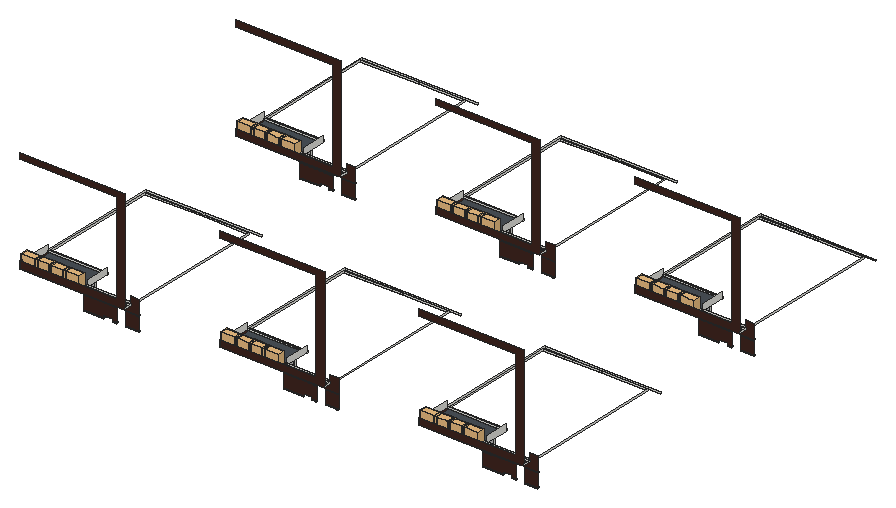
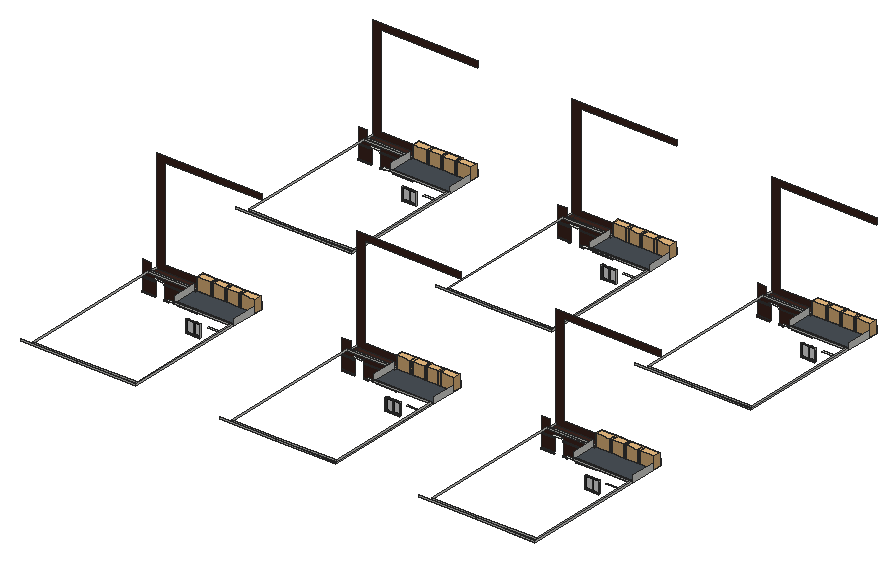
# SketchUp Ruby script. Lengths in inches.
U = 1.inch
M = Sketchup.active_model
def pt(a) = Geom::Point3d.new(a.map { |v| v * U })
def face(e, loops, mat)
  f = e.add_face(loops[0].map { |a| pt(a) })
  loops[1..].each { |l| e.add_face(l.map { |a| pt(a) }).erase! }
  f.material = f.back_material = mat if mat
  f
end
# faces: each face lists its corners as indices into pts; further lists are holes
def faces(e, pts, list, mat = nil) = list.each { |f| face(e, (f[0].is_a?(Array) ? f : [f]).map { |l| l.map { |i| pts[i] } }, mat) }
# xy, xz, yz: faces in a plane at the given z, y or x. An outline is a flat list of corners, or four numbers for a rectangle; further outlines are holes
def ring(l) = l.size == 4 ? [[l[0], l[1]], [l[2], l[1]], [l[2], l[3]], [l[0], l[3]]] : l.each_slice(2).to_a
def flat(e, list, mat, &to3) = list.each { |f| face(e, (f[0].is_a?(Array) ? f : [f]).map { |l| ring(l).map { |u, v| to3.(u, v) } }, mat) }
def xy(e, z, list, mat = nil) = flat(e, list, mat) { |x, y| [x, y, z] }
def xz(e, y, list, mat = nil) = flat(e, list, mat) { |x, z| [x, y, z] }
def yz(e, x, list, mat = nil) = flat(e, list, mat) { |y, z| [x, y, z] }
def lines(e, pts, list) = list.each { |a, b| e.add_line(pt(pts[a]), pt(pts[b])) }
# prism: a flat outline (further loops are holes) pulled along v
def prism(e, loops, v, mat = nil)
  f = face(e, loops, mat); d = Geom::Vector3d.new(v.map { |x| x * U })
  f.pushpull(f.normal.samedirection?(d) ? d.length : -d.length)
end
def box(e, o, s, mat = nil) = prism(e, [[o, [o[0] + s[0], o[1], o[2]], [o[0] + s[0], o[1] + s[1], o[2]], [o[0], o[1] + s[1], o[2]]]], [0, 0, s[2]], mat)
def at(x, y, z, deg = 0) = Geom::Transformation.translation(pt([x, y, z])) * Geom::Transformation.rotation(ORIGIN, Z_AXIS, deg.degrees)
def axes(o, x, y, z) = Geom::Transformation.new([*x, 0, *y, 0, *z, 0, *pt(o).to_a, 1])
def part(name) = M.definitions.add(name)
# library, detail: a bought-in or finely detailed component or shape, given as its bounding box
def library(name, o, s) = part(name).tap { |d| box(d.entities, o, s) }
def detail(e, o, s) = box(e.add_group.entities, o, s)
def put(e, d, t, mat = nil) = e.add_instance(d, t).tap { |i| i.material = mat if mat }
def group(e, t, mat = nil) = e.add_group.tap { |g| g.transformation = t; g.material = mat if mat }.entities
root = M.entities
M.materials.add("Glass_Tinted_Gray").color = [0, 0, 0]
M.materials["Glass_Tinted_Gray"].alpha = 0.125
M.materials.add("[0043_SaddleBrown]").color = [63, 38, 31]
M.materials.add("[0135_DarkGray]").color = [81, 81, 81]
M.materials.add("[Formica Blue]").color = [73, 80, 86]
M.materials.add("[Mirror 02]").color = [229, 229, 229]
M.materials.add("[Terrazzo Light Blue]").color = [196, 214, 227]
c1 = part("PENTEK_RP Fineline 50S_Sliding_DoorCase_E1")
box(c1.entities,[0,0,0],[1.51,3.66,99.27],"[0135_DarkGray]")
c2 = part("PENTEK_RP Fineline 50S_SlidingDooe_Case_E2")
box(c2.entities,[0,0,0],[96.25,3.66,1.51],"[0135_DarkGray]")
c3 = part("pentek_RP Fineline 50S_SlidingDoor_Case")
put(c3.entities,c1,at(97.76,0,0))
put(c3.entities,c2,at(1.51,0,0))
put(c3.entities,c1,at(0,0,0))
put(c3.entities,c2,at(1.51,0,97.76))
c4 = part("PENTEK_RP Fineline 50S_SlidingDoor_GlazingBead_2")
box(c4.entities,[0,0,0],[0.56,0.59,94.39],"[0135_DarkGray]")
c5 = part("PENTEK_RP Fineline 50S_SlidingDoor_Glass")
box(c5.entities,[0,0,0],[46.58,0.16,94.39],"Glass_Tinted_Gray")
c6 = part("PENTEK_RP Fineline 50S_SlidingDoor_GlazingBead")
box(c6.entities,[0,0,0],[45.47,0.59,0.56],"[0135_DarkGray]")
c7 = part("PENTEK_RP Fineline 50S_SlidingDoor_Leaf_E1")
xy(c7.entities,0,[[0,0,0.93,1.97],[0.93,1.57,1.49,1.97]],"[0135_DarkGray]")
xy(c7.entities,96.25,[[0,0,0.93,0,0.93,1.57,1.49,1.57,1.49,1.97,0,1.97]],"[0135_DarkGray]")
xz(c7.entities,0,[[0,0,0.93,96.25]],"[0135_DarkGray]")
xz(c7.entities,1.57,[[0.93,0,1.49,95.32],[0.93,95.32,1.49,96.25]],"[0135_DarkGray]")
xz(c7.entities,1.97,[[0,0,1.49,96.25]],"[0135_DarkGray]")
yz(c7.entities,0,[[0,0,1.97,96.25]],"[0135_DarkGray]")
yz(c7.entities,0.93,[[0,0,1.57,0.93],[0,0.93,1.57,95.32],[0,95.32,1.57,96.25]],"[0135_DarkGray]")
yz(c7.entities,1.49,[[1.57,0,1.97,95.32],[1.57,95.32,1.97,96.25]],"[0135_DarkGray]")
c8 = part("PENTEK_RP Fineline 50S_SlidingDoor_Leaf_E2")
xy(c8.entities,0,[[0,0,0,1.57,0.56,1.57,0.56,1.97,46.02,1.97,46.02,1.57,46.58,1.57,46.58,0]],"[0135_DarkGray]")
xy(c8.entities,0.93,[[0,0,46.58,1.57]],"[0135_DarkGray]")
xy(c8.entities,1.49,[[0.56,1.57,46.02,1.97]],"[0135_DarkGray]")
xz(c8.entities,0,[[0,0,46.58,0.93]],"[0135_DarkGray]")
xz(c8.entities,1.57,[[0,0,0.56,0.93],[46.02,0,46.58,0.93],[0.56,0.93,46.02,1.49]],"[0135_DarkGray]")
xz(c8.entities,1.97,[[0.56,0,46.02,1.49]],"[0135_DarkGray]")
yz(c8.entities,0,[[0,0,1.57,0.93]],"[0135_DarkGray]")
yz(c8.entities,0.56,[[1.57,0,1.97,0.93],[1.57,0.93,1.97,1.49]],"[0135_DarkGray]")
yz(c8.entities,46.02,[[1.57,0,1.97,0.93],[1.57,0.93,1.97,1.49]],"[0135_DarkGray]")
yz(c8.entities,46.58,[[0,0,1.57,0.93]],"[0135_DarkGray]")
c9 = part("PENTEK_RP Fineline S_SlidingDoor_Leaf1")
put(c9.entities,c4,at(0.93,0,0.93))
put(c9.entities,c4,at(46.96,0,0.93))
put(c9.entities,c5,at(1.49,1.42,0.93))
put(c9.entities,c6,at(1.49,0,0.93))
put(c9.entities,c5,at(1.49,0.59,0.93),"[Terrazzo Light Blue]")
put(c9.entities,c7,at(0,0,0))
put(c9.entities,c7,axes([48.44,0,0],[-1,0,0],[0,1,0],[0,0,1]))
put(c9.entities,c8,axes([0.93,0,96.25],[1,0,0],[0,1,0],[0,0,-1]))
put(c9.entities,c8,at(0.93,0,0))
put(c9.entities,c6,at(1.49,0,94.77))
c10 = part("PENTEK_RP Fineline 50S_SlidingDoor_Leaf2")
put(c10.entities,c5,at(1.49,1.42,0.93))
put(c10.entities,c6,at(1.49,0,94.77))
put(c10.entities,c4,at(46.96,0,0.93))
put(c10.entities,c5,at(1.49,0.59,0.93),"[Mirror 02]")
put(c10.entities,c4,at(0.93,0,0.93))
put(c10.entities,c7,at(0,0,0))
put(c10.entities,c7,axes([48.44,0,0],[-1,0,0],[0,1,0],[0,0,1]))
put(c10.entities,c6,at(1.49,0,0.93))
put(c10.entities,c8,axes([0.93,0,96.25],[1,0,0],[0,1,0],[0,0,-1]))
put(c10.entities,c8,at(0.93,0,0))
c11 = part("PENTEK - Slimmest Steel Sliding Door / Window\#1")
put(c11.entities,c3,at(0,-1.88,-0.09))
put(c11.entities,c9,at(1.51,-2.27,1.42))
put(c11.entities,c10,at(49.32,-0.3,1.42))
c12 = library("Group13",[-203.48,36.63,0],[29.68,67.31,50.64])
xy(root,298.0625,[[258.09,535.375,309.84,540.48],[982.53,535.375,1034.28,540.48],[1706.96,535.375,1758.71,540.48],[258.09,1515.73,309.84,1520.83],[982.53,1515.73,1034.28,1520.83],
  [1706.96,1515.73,1758.71,1520.83]])
xy(root,303,[[348.1875,438.72,419.76,441.04],[451.01,438.72,467.3,441.04],[1072.625,438.72,1144.2,441.04],[1175.45,438.72,1191.74,441.04],[1797.0625,438.72,1868.64,441.04],
  [1899.89,438.72,1916.17,441.04],[500.42,438.73,547.05,441.04],[1224.86,438.73,1271.49,441.04],[1949.3,438.73,1995.93,441.04],[348.1875,1419.07,419.76,1421.39],
  [451.01,1419.07,467.3,1421.39],[1072.625,1419.07,1144.2,1421.39],[1175.45,1419.07,1191.74,1421.39],[1797.0625,1419.07,1868.64,1421.39],[1899.89,1419.07,1916.17,1421.39],
  [500.42,1419.08,547.05,1421.39],[1224.86,1419.08,1271.49,1421.39],[1949.3,1419.08,1995.93,1421.39]])
xy(root,306.15,[[348.1875,438.72,419.76,441.04],[1072.625,438.72,1144.2,441.04],[1797.0625,438.72,1868.64,441.04],[348.1875,1419.07,348.1875,1421.39,419.76,1421.39,419.76,1419.08],[1072.625,1419.07,1072.625,1421.39,1144.2,1421.39,1144.2,1419.08],
  [1797.0625,1419.07,1797.0625,1421.39,1868.64,1421.39,1868.64,1419.08]])
xy(root,306.7,[[547.05,438.72,500.42,438.73,500.42,441.04,547.05,441.04],[1271.49,438.72,1224.86,438.73,1224.86,441.04,1271.49,441.04],[1995.93,438.72,1949.3,438.73,1949.3,441.04,1995.93,441.04],[547.05,1419.07,500.42,1419.08,500.42,1421.39,547.05,1421.39],[1271.49,1419.07,1224.86,1419.08,1224.86,1421.39,1271.49,1421.39],
  [1995.93,1419.07,1949.3,1419.08,1949.3,1421.39,1995.93,1421.39]])
xy(root,306.93,[[451.01,438.72,467.3,441.04],[1175.45,438.72,1191.74,441.04],[1899.89,438.72,1916.17,441.04],[451.01,1419.07,467.3,1421.39],[1175.45,1419.07,1191.74,1421.39],
  [1899.89,1419.07,1916.17,1421.39]])
xy(root,312.4,[[419.76,438.72,451.01,447.84],[1144.2,438.72,1175.45,447.84],[1868.64,438.72,1899.89,447.84],[419.76,1419.07,451.01,1428.19],[1144.2,1419.07,1175.45,1428.19],
  [1868.64,1419.07,1899.89,1428.19]])
xy(root,342.25,[[183.3,535.375,231.3,540.48],[258.09,535.375,309.84,540.48],[907.74,535.375,955.74,540.48],[982.53,535.375,1034.28,540.48],[1632.17,535.375,1680.17,540.48],
  [1706.96,535.375,1758.71,540.48],[183.3,1515.73,231.3,1520.83],[258.09,1515.73,309.84,1520.83],[907.74,1515.73,955.74,1520.83],[982.53,1515.73,1034.28,1520.83],
  [1632.17,1515.73,1680.17,1520.83],[1706.96,1515.73,1758.71,1520.83]])
xy(root,354.05,[[348.1875,438.72,467.3,441.04],[1072.625,438.72,1191.74,441.04],[1797.0625,438.72,1916.17,441.04],[348.1875,1419.07,467.3,1421.39],[1072.625,1419.07,1191.74,1421.39],
  [1797.0625,1419.07,1916.17,1421.39]])
xy(root,354.27,[[547.05,438.72,547.05,441.04,500.42,441.04,500.42,438.73],[1271.49,438.72,1271.49,441.04,1224.86,441.04,1224.86,438.73],[1995.93,438.72,1995.93,441.04,1949.3,441.04,1949.3,438.73],[547.05,1419.07,547.05,1421.39,500.42,1421.39,500.42,1419.08],[1271.49,1419.07,1271.49,1421.39,1224.86,1421.39,1224.86,1419.08],
  [1995.93,1419.07,1995.93,1421.39,1949.3,1421.39,1949.3,1419.08]])
xy(root,355.72,[[348.1875,438.72,467.3,441.04],[1072.625,438.72,1191.74,441.04],[1797.0625,438.72,1916.17,441.04],[348.1875,1419.07,467.3,1421.39],[1072.625,1419.07,1191.74,1421.39],
  [1797.0625,1419.07,1916.17,1421.39]])
xy(root,357.3,[[500.42,438.73,547.05,441.04],[1224.86,438.73,1271.49,441.04],[1949.3,438.73,1995.93,441.04],[500.42,1419.08,547.05,1421.39],[1224.86,1419.08,1271.49,1421.39],
  [1949.3,1419.08,1995.93,1421.39]])
xy(root,365.23,[[467.3,438.72,500.42,447.84],[1191.74,438.72,1224.86,447.84],[1916.17,438.72,1949.3,447.84],[467.3,1419.07,500.42,1428.19],[1191.74,1419.07,1224.86,1428.19],
  [1916.17,1419.07,1949.3,1428.19]])
xy(root,378.25,[[348.1875,438.72,353.97,447.84],[1072.625,438.72,1078.41,447.84],[1797.0625,438.72,1802.84,447.84],[137.5,535.375,137.5,980.35,353.97,980.35,353.97,971.23,144.84,965.96,144.84,540.48,353.97,540.48,353.97,535.375],[861.9375,535.375,861.9375,980.35,1078.41,980.35,1078.41,971.23,869.28,965.96,869.28,540.48,1078.41,540.48,1078.41,535.375],
  [1586.375,535.375,1586.375,980.35,1802.84,980.35,1802.84,971.23,1593.72,965.96,1593.72,540.48,1802.84,540.48,1802.84,535.375],[348.1875,1419.07,353.97,1428.19],[1072.625,1419.07,1078.41,1428.19],[1797.0625,1419.07,1802.84,1428.19],[137.5,1515.73,137.5,1960.7,353.97,1960.7,353.97,1951.58,144.84,1946.3125,144.84,1520.83,353.97,1520.83,353.97,1515.73],
  [861.9375,1515.73,861.9375,1960.7,1078.41,1960.7,1078.41,1951.58,869.28,1946.3125,869.28,1520.83,1078.41,1520.83,1078.41,1515.73],[1586.375,1515.73,1586.375,1960.7,1802.84,1960.7,1802.84,1951.58,1593.72,1946.3125,1593.72,1520.83,1802.84,1520.83,1802.84,1515.73]])
xy(root,378.25,[[137.5,412.04,137.5,535.375,144.5,535.375,144.5,438.72,504.5,438.72,504.5,412.04],[504.5,412.04,517.3125,438.72],[861.9375,412.04,861.9375,535.375,868.9375,535.375,868.9375,438.72,1228.9375,438.72,1228.9375,412.04],[1228.9375,412.04,1241.75,438.72],[1586.375,412.04,1586.375,535.375,1593.375,535.375,1593.375,438.72,1953.375,438.72,1953.375,412.04],
  [1953.375,412.04,1966.1875,438.72],[137.5,1392.39,137.5,1515.73,144.5,1515.73,144.5,1419.07,504.5,1419.07,504.5,1392.39],[504.5,1392.39,517.3125,1419.07],[861.9375,1392.39,861.9375,1515.73,868.9375,1515.73,868.9375,1419.07,1228.9375,1419.07,1228.9375,1392.39],[1228.9375,1392.39,1241.75,1419.07],
  [1586.375,1392.39,1586.375,1515.73,1593.375,1515.73,1593.375,1419.07,1953.375,1419.07,1953.375,1392.39],[1953.375,1392.39,1966.1875,1419.07]],"[0043_SaddleBrown]")
xy(root,378.25,[[144.5,438.72,144.5,535.375,353.97,535.375,353.97,447.84,348.1875,447.84,348.1875,438.72],[868.9375,438.72,868.9375,535.375,1078.41,535.375,1078.41,447.84,1072.625,447.84,1072.625,438.72],[1593.375,438.72,1593.375,535.375,1802.84,535.375,1802.84,447.84,1797.0625,447.84,1797.0625,438.72],[144.5,1419.07,144.5,1515.73,353.97,1515.73,353.97,1428.19,348.1875,1428.19,348.1875,1419.07],[868.9375,1419.07,868.9375,1515.73,1078.41,1515.73,1078.41,1428.19,1072.625,1428.19,1072.625,1419.07],
  [1593.375,1419.07,1593.375,1515.73,1802.84,1515.73,1802.84,1428.19,1797.0625,1428.19,1797.0625,1419.07]],"[Formica Blue]")
xz(root,412.04,[[137.5,378.25,517.3125,378.25,517.3125,755.5,137.5,755.5,137.5,733.125,487.0625,733.125,487.0625,401.6875,137.5,401.6875],[861.9375,378.25,1241.75,378.25,1241.75,755.5,861.9375,755.5,861.9375,733.125,1211.5,733.125,1211.5,401.6875,861.9375,401.6875],[1586.375,378.25,1966.1875,378.25,1966.1875,755.5,1586.375,755.5,1586.375,733.125,1935.9375,733.125,1935.9375,401.6875,1586.375,401.6875]],"[0043_SaddleBrown]")
xz(root,438.72,[[348.1875,378.25,353.97,384.25],[353.97,378.25,504.5,384.25],[504.5,378.25,517.3125,384.25],[1072.625,378.25,1078.41,384.25],[1078.41,378.25,1228.9375,384.25],
  [1228.9375,378.25,1241.75,384.25],[1797.0625,378.25,1802.84,384.25],[1802.84,378.25,1953.375,384.25],[1953.375,378.25,1966.1875,384.25]])
xz(root,438.72,[[348.1875,306.15,419.76,306.15,419.76,312.4,451.01,312.4,451.01,306.93,467.3,306.93,467.3,354.05,348.1875,354.05],[1072.625,306.15,1144.2,306.15,1144.2,312.4,1175.45,312.4,1175.45,306.93,1191.74,306.93,1191.74,354.05,1072.625,354.05],[1797.0625,306.15,1868.64,306.15,1868.64,312.4,1899.89,312.4,1899.89,306.93,1916.17,306.93,1916.17,354.05,1797.0625,354.05]],"[0043_SaddleBrown]")
xz(root,441.04,[[348.1875,303,419.76,306.15],[451.01,303,467.3,306.93],[500.42,303,547.05,306.7],[1072.625,303,1144.2,306.15],[1175.45,303,1191.74,306.93],
  [1224.86,303,1271.49,306.7],[1797.0625,303,1868.64,306.15],[1899.89,303,1916.17,306.93],[1949.3,303,1995.93,306.7],[348.1875,354.05,467.3,355.72],
  [1072.625,354.05,1191.74,355.72],[1797.0625,354.05,1916.17,355.72],[500.42,354.27,547.05,357.3],[1224.86,354.27,1271.49,357.3],[1949.3,354.27,1995.93,357.3]],"[0043_SaddleBrown]")
xz(root,447.84,[[348.1875,378.25,353.97,384.25],[353.97,378.25,521.63,384.25],[1072.625,378.25,1078.41,384.25],[1078.41,378.25,1246.07,384.25],[1797.0625,378.25,1802.84,384.25],
  [1802.84,378.25,1970.51,384.25]])
xz(root,535.375,[[137.5,378.25,353.97,384.25],[861.9375,378.25,1078.41,384.25],[1586.375,378.25,1802.84,384.25]])
xz(root,540.48,[[144.84,378.25,353.97,384.25],[869.28,378.25,1078.41,384.25],[1593.72,378.25,1802.84,384.25]])
xz(root,971.23,[[353.97,378.25,521.63,384.25],[1078.41,378.25,1246.07,384.25],[1802.84,378.25,1970.51,384.25]])
xz(root,980.35,[[137.5,378.25,353.97,384.25],[353.97,378.25,558.625,384.25],[861.9375,378.25,1078.41,384.25],[1078.41,378.25,1283.0625,384.25],[1586.375,378.25,1802.84,384.25],
  [1802.84,378.25,2007.5,384.25]])
xz(root,1392.39,[[137.5,378.25,517.3125,378.25,517.3125,755.5,137.5,755.5,137.5,733.125,487.0625,733.125,487.0625,401.6875,137.5,401.6875],[861.9375,378.25,1241.75,378.25,1241.75,755.5,861.9375,755.5,861.9375,733.125,1211.5,733.125,1211.5,401.6875,861.9375,401.6875],[1586.375,378.25,1966.1875,378.25,1966.1875,755.5,1586.375,755.5,1586.375,733.125,1935.9375,733.125,1935.9375,401.6875,1586.375,401.6875]],"[0043_SaddleBrown]")
xz(root,1419.07,[[348.1875,378.25,353.97,384.25],[353.97,378.25,504.5,384.25],[504.5,378.25,517.3125,384.25],[1072.625,378.25,1078.41,384.25],[1078.41,378.25,1228.9375,384.25],
  [1228.9375,378.25,1241.75,384.25],[1797.0625,378.25,1802.84,384.25],[1802.84,378.25,1953.375,384.25],[1953.375,378.25,1966.1875,384.25]])
xz(root,1421.39,[[348.1875,303,419.76,306.15],[451.01,303,467.3,306.93],[500.42,303,547.05,306.7],[1072.625,303,1144.2,306.15],[1175.45,303,1191.74,306.93],
  [1224.86,303,1271.49,306.7],[1797.0625,303,1868.64,306.15],[1899.89,303,1916.17,306.93],[1949.3,303,1995.93,306.7],[348.1875,354.05,467.3,355.72],
  [1072.625,354.05,1191.74,355.72],[1797.0625,354.05,1916.17,355.72],[500.42,354.27,547.05,357.3],[1224.86,354.27,1271.49,357.3],[1949.3,354.27,1995.93,357.3]],"[0043_SaddleBrown]")
xz(root,1428.19,[[348.1875,378.25,353.97,384.25],[353.97,378.25,521.63,384.25],[1072.625,378.25,1078.41,384.25],[1078.41,378.25,1246.07,384.25],[1797.0625,378.25,1802.84,384.25],
  [1802.84,378.25,1970.51,384.25]])
xz(root,1515.73,[[137.5,378.25,353.97,384.25],[861.9375,378.25,1078.41,384.25],[1586.375,378.25,1802.84,384.25]])
xz(root,1520.83,[[144.84,378.25,353.97,384.25],[869.28,378.25,1078.41,384.25],[1593.72,378.25,1802.84,384.25]])
xz(root,1951.58,[[353.97,378.25,521.63,384.25],[1078.41,378.25,1246.07,384.25],[1802.84,378.25,1970.51,384.25]])
xz(root,1960.7,[[137.5,378.25,353.97,384.25],[353.97,378.25,558.625,384.25],[861.9375,378.25,1078.41,384.25],[1078.41,378.25,1283.0625,384.25],[1586.375,378.25,1802.84,384.25],
  [1802.84,378.25,2007.5,384.25]])
yz(root,137.5,[[412.04,378.25,535.375,401.6875],[535.375,378.25,980.35,384.25],[1392.39,378.25,1515.73,401.6875],[1515.73,378.25,1960.7,384.25]])
yz(root,144.84,[[540.48,378.25,965.96,384.25],[1520.83,378.25,1946.3125,384.25]])
yz(root,258.09,[[535.375,298.0625,540.48,342.25],[1515.73,298.0625,1520.83,342.25]])
yz(root,309.84,[[535.375,298.0625,540.48,342.25],[1515.73,298.0625,1520.83,342.25]])
yz(root,348.1875,[[438.72,378.25,447.84,384.25],[1419.07,378.25,1428.19,384.25]])
yz(root,353.97,[[438.72,378.25,447.84,384.25],[447.84,378.25,535.375,401.6875],[535.375,378.25,540.48,384.25],[971.23,378.25,980.35,384.25],[1419.07,378.25,1428.19,384.25],
  [1428.19,378.25,1515.73,401.6875],[1515.73,378.25,1520.83,384.25],[1951.58,378.25,1960.7,384.25]])
yz(root,517.3125,[[412.04,378.25,438.72,384.25],[1392.39,378.25,1419.07,384.25]])
yz(root,521.63,[[447.84,378.25,971.23,384.25],[1428.19,378.25,1951.58,384.25]])
yz(root,861.9375,[[412.04,378.25,535.375,401.6875],[535.375,378.25,980.35,384.25],[1392.39,378.25,1515.73,401.6875],[1515.73,378.25,1960.7,384.25]])
yz(root,869.28,[[540.48,378.25,965.96,384.25],[1520.83,378.25,1946.3125,384.25]])
yz(root,982.53,[[535.375,298.0625,540.48,342.25],[1515.73,298.0625,1520.83,342.25]])
yz(root,1034.28,[[535.375,298.0625,540.48,342.25],[1515.73,298.0625,1520.83,342.25]])
yz(root,1072.625,[[438.72,378.25,447.84,384.25],[1419.07,378.25,1428.19,384.25]])
yz(root,1078.41,[[438.72,378.25,447.84,384.25],[447.84,378.25,535.375,401.6875],[535.375,378.25,540.48,384.25],[971.23,378.25,980.35,384.25],[1419.07,378.25,1428.19,384.25],
  [1428.19,378.25,1515.73,401.6875],[1515.73,378.25,1520.83,384.25],[1951.58,378.25,1960.7,384.25]])
yz(root,1241.75,[[412.04,378.25,438.72,384.25],[1392.39,378.25,1419.07,384.25]])
yz(root,1246.07,[[447.84,378.25,971.23,384.25],[1428.19,378.25,1951.58,384.25]])
yz(root,1586.375,[[412.04,378.25,535.375,401.6875],[535.375,378.25,980.35,384.25],[1392.39,378.25,1515.73,401.6875],[1515.73,378.25,1960.7,384.25]])
yz(root,1593.72,[[540.48,378.25,965.96,384.25],[1520.83,378.25,1946.3125,384.25]])
yz(root,1706.96,[[535.375,298.0625,540.48,342.25],[1515.73,298.0625,1520.83,342.25]])
yz(root,1758.71,[[535.375,298.0625,540.48,342.25],[1515.73,298.0625,1520.83,342.25]])
yz(root,1797.0625,[[438.72,378.25,447.84,384.25],[1419.07,378.25,1428.19,384.25]])
yz(root,1802.84,[[438.72,378.25,447.84,384.25],[447.84,378.25,535.375,401.6875],[535.375,378.25,540.48,384.25],[971.23,378.25,980.35,384.25],[1419.07,378.25,1428.19,384.25],
  [1428.19,378.25,1515.73,401.6875],[1515.73,378.25,1520.83,384.25],[1951.58,378.25,1960.7,384.25]])
yz(root,1966.1875,[[412.04,378.25,438.72,384.25],[1392.39,378.25,1419.07,384.25]])
yz(root,1970.51,[[447.84,378.25,971.23,384.25],[1428.19,378.25,1951.58,384.25]])
p = [[451.01,1419.07,312.4],[451.01,1419.07,306.93],[467.3,1419.07,306.93],[467.3,1419.07,354.05],[348.1875,1419.07,354.05],[348.1875,1419.07,306.15],
  [419.76,1419.08,306.15],[419.76,1419.07,312.4],[1175.45,1419.07,312.4],[1175.45,1419.07,306.93],[1191.74,1419.07,306.93],[1191.74,1419.07,354.05],
  [1072.625,1419.07,354.05],[1072.625,1419.07,306.15],[1144.2,1419.08,306.15],[1144.2,1419.07,312.4],[1899.89,1419.07,312.4],[1899.89,1419.07,306.93],
  [1916.17,1419.07,306.93],[1916.17,1419.07,354.05],[1797.0625,1419.07,354.05],[1797.0625,1419.07,306.15],[1868.64,1419.08,306.15],[1868.64,1419.07,312.4],
  [500.42,438.73,354.27],[500.42,438.73,306.7],[547.05,438.72,306.7],[547.05,438.72,354.27],[1224.86,438.73,354.27],[1224.86,438.73,306.7],
  [1271.49,438.72,306.7],[1271.49,438.72,354.27],[1949.3,438.73,354.27],[1949.3,438.73,306.7],[1995.93,438.72,306.7],[1995.93,438.72,354.27],
  [500.42,1419.08,354.27],[500.42,1419.08,306.7],[547.05,1419.07,306.7],[547.05,1419.07,354.27],[1224.86,1419.08,354.27],[1224.86,1419.08,306.7],
  [1271.49,1419.07,306.7],[1271.49,1419.07,354.27],[1949.3,1419.08,354.27],[1949.3,1419.08,306.7],[1995.93,1419.07,306.7],[1995.93,1419.07,354.27],
  [547.05,438.73,357.3],[547.05,438.73,409.48],[517.3125,438.73,409.48],[517.3125,438.72,384.25],[517.3125,438.72,378.25],[504.5,438.72,378.25],
  [353.97,438.72,378.25],[348.1875,438.72,378.25],[348.1875,438.72,355.72],[467.3,438.72,355.72],[467.3,438.72,365.23],[500.42,438.72,365.23],
  [500.42,438.73,357.3],[1271.49,438.73,357.3],[1271.49,438.73,409.48],[1241.75,438.73,409.48],[1241.75,438.72,384.25],[1241.75,438.72,378.25],
  [1228.9375,438.72,378.25],[1078.41,438.72,378.25],[1072.625,438.72,378.25],[1072.625,438.72,355.72],[1191.74,438.72,355.72],[1191.74,438.72,365.23],
  [1224.86,438.72,365.23],[1224.86,438.73,357.3],[1995.93,438.73,357.3],[1995.93,438.73,409.48],[1966.1875,438.73,409.48],[1966.1875,438.72,384.25],
  [1966.1875,438.72,378.25],[1953.375,438.72,378.25],[1802.84,438.72,378.25],[1797.0625,438.72,378.25],[1797.0625,438.72,355.72],[1916.17,438.72,355.72],
  [1916.17,438.72,365.23],[1949.3,438.72,365.23],[1949.3,438.73,357.3],[547.05,1419.08,357.3],[547.05,1419.08,409.48],[517.3125,1419.08,409.48],
  [517.3125,1419.07,384.25],[517.3125,1419.07,378.25],[504.5,1419.07,378.25],[353.97,1419.07,378.25],[348.1875,1419.07,378.25],[348.1875,1419.07,355.72],
  [467.3,1419.07,355.72],[467.3,1419.07,365.23],[500.42,1419.07,365.23],[500.42,1419.08,357.3],[1271.49,1419.08,357.3],[1271.49,1419.08,409.48],
  [1241.75,1419.08,409.48],[1241.75,1419.07,384.25],[1241.75,1419.07,378.25],[1228.9375,1419.07,378.25],[1078.41,1419.07,378.25],[1072.625,1419.07,378.25],
  [1072.625,1419.07,355.72],[1191.74,1419.07,355.72],[1191.74,1419.07,365.23],[1224.86,1419.07,365.23],[1224.86,1419.08,357.3],[1995.93,1419.08,357.3],
  [1995.93,1419.08,409.48],[1966.1875,1419.08,409.48],[1966.1875,1419.07,384.25],[1966.1875,1419.07,378.25],[1953.375,1419.07,378.25],[1802.84,1419.07,378.25],
  [1797.0625,1419.07,378.25],[1797.0625,1419.07,355.72],[1916.17,1419.07,355.72],[1916.17,1419.07,365.23],[1949.3,1419.07,365.23],[1949.3,1419.08,357.3],
  [144.84,965.96,378.25],[353.97,971.23,378.25],[353.97,971.23,384.25],[144.84,965.96,384.25],[869.28,965.96,378.25],[1078.41,971.23,378.25],
  [1078.41,971.23,384.25],[869.28,965.96,384.25],[1593.72,965.96,378.25],[1802.84,971.23,378.25],[1802.84,971.23,384.25],[1593.72,965.96,384.25],
  [144.84,1946.3125,378.25],[353.97,1951.58,378.25],[353.97,1951.58,384.25],[144.84,1946.3125,384.25],[869.28,1946.3125,378.25],[1078.41,1951.58,378.25],
  [1078.41,1951.58,384.25],[869.28,1946.3125,384.25],[1593.72,1946.3125,378.25],[1802.84,1951.58,378.25],[1802.84,1951.58,384.25],[1593.72,1946.3125,384.25]]
faces(root,p,[[0,1,2,3,4,5,6,7],[8,9,10,11,12,13,14,15],[16,17,18,19,20,21,22,23],[24,25,26,27],[28,29,30,31],[32,33,34,35],[36,37,38,39],[40,41,42,43],
  [44,45,46,47],[48,49,50,51,52,53,54,55,56,57,58,59,60],[61,62,63,64,65,66,67,68,69,70,71,72,73],[74,75,76,77,78,79,80,81,82,83,84,85,86],[87,88,89,90,91,92,93,94,95,96,97,98,99],[100,101,102,103,104,105,106,107,108,109,110,111,112],[113,114,115,116,117,118,119,120,121,122,123,124,125]],"[0043_SaddleBrown]")
faces(root,p,[[126,127,128,129],[130,131,132,133],[134,135,136,137],[138,139,140,141],[142,143,144,145],[146,147,148,149]])
put(root,c11,axes([258.09,1515.73,298.0625],[0.52129,0,0],[0,0.44,0],[0,0,0.44603]))
put(root,c11,axes([1706.96,1515.73,298.0625],[0.52129,0,0],[0,0.44,0],[0,0,0.44603]))
put(root,c11,axes([982.53,1515.73,298.0625],[0.52129,0,0],[0,0.44,0],[0,0,0.44603]))
put(root,c11,axes([982.53,535.375,298.0625],[0.52129,0,0],[0,0.44,0],[0,0,0.44603]))
put(root,c11,axes([1706.96,535.375,298.0625],[0.52129,0,0],[0,0.44,0],[0,0,0.44603]))
put(root,c11,axes([258.09,535.375,298.0625],[0.52129,0,0],[0,0.44,0],[0,0,0.44603]))
put(root,c12,axes([879.59,1245.5,379.98],[0,-0.8723,0],[0.8723,0,0],[0,0,0.8723]))
put(root,c12,axes([930.96,1245.5,379.98],[0,-0.8723,0],[0.8723,0,0],[0,0,0.8723]))
put(root,c12,axes([980.65,1245.5,379.98],[0,-0.8723,0],[0.8723,0,0],[0,0,0.8723]))
put(root,c12,axes([829.65,1245.5,379.98],[0,-0.8723,0],[0.8723,0,0],[0,0,0.8723]))
put(root,c12,axes([155.15,1245.5,379.98],[0,-0.8723,0],[0.8723,0,0],[0,0,0.8723]))
put(root,c12,axes([256.21,1245.5,379.98],[0,-0.8723,0],[0.8723,0,0],[0,0,0.8723]))
put(root,c12,axes([206.53,1245.5,379.98],[0,-0.8723,0],[0.8723,0,0],[0,0,0.8723]))
put(root,c12,axes([1705.09,1245.5,379.98],[0,-0.8723,0],[0.8723,0,0],[0,0,0.8723]))
put(root,c12,axes([105.21,1245.5,379.98],[0,-0.8723,0],[0.8723,0,0],[0,0,0.8723]))
put(root,c12,axes([1554.09,1245.5,379.98],[0,-0.8723,0],[0.8723,0,0],[0,0,0.8723]))
put(root,c12,axes([1604.03,1245.5,379.98],[0,-0.8723,0],[0.8723,0,0],[0,0,0.8723]))
put(root,c12,axes([1655.4,1245.5,379.98],[0,-0.8723,0],[0.8723,0,0],[0,0,0.8723]))
put(root,c12,axes([829.65,265.15,379.98],[0,-0.8723,0],[0.8723,0,0],[0,0,0.8723]))
put(root,c12,axes([879.59,265.15,379.98],[0,-0.8723,0],[0.8723,0,0],[0,0,0.8723]))
put(root,c12,axes([930.96,265.15,379.98],[0,-0.8723,0],[0.8723,0,0],[0,0,0.8723]))
put(root,c12,axes([980.65,265.15,379.98],[0,-0.8723,0],[0.8723,0,0],[0,0,0.8723]))
put(root,c12,axes([1554.09,265.15,379.98],[0,-0.8723,0],[0.8723,0,0],[0,0,0.8723]))
put(root,c12,axes([1604.03,265.15,379.98],[0,-0.8723,0],[0.8723,0,0],[0,0,0.8723]))
put(root,c12,axes([1655.4,265.15,379.98],[0,-0.8723,0],[0.8723,0,0],[0,0,0.8723]))
put(root,c12,axes([1705.09,265.15,379.98],[0,-0.8723,0],[0.8723,0,0],[0,0,0.8723]))
put(root,c12,axes([206.53,265.15,379.98],[0,-0.8723,0],[0.8723,0,0],[0,0,0.8723]))
put(root,c12,axes([256.21,265.15,379.98],[0,-0.8723,0],[0.8723,0,0],[0,0,0.8723]))
put(root,c12,axes([105.21,265.15,379.98],[0,-0.8723,0],[0.8723,0,0],[0,0,0.8723]))
put(root,c12,axes([155.15,265.15,379.98],[0,-0.8723,0],[0.8723,0,0],[0,0,0.8723]))
